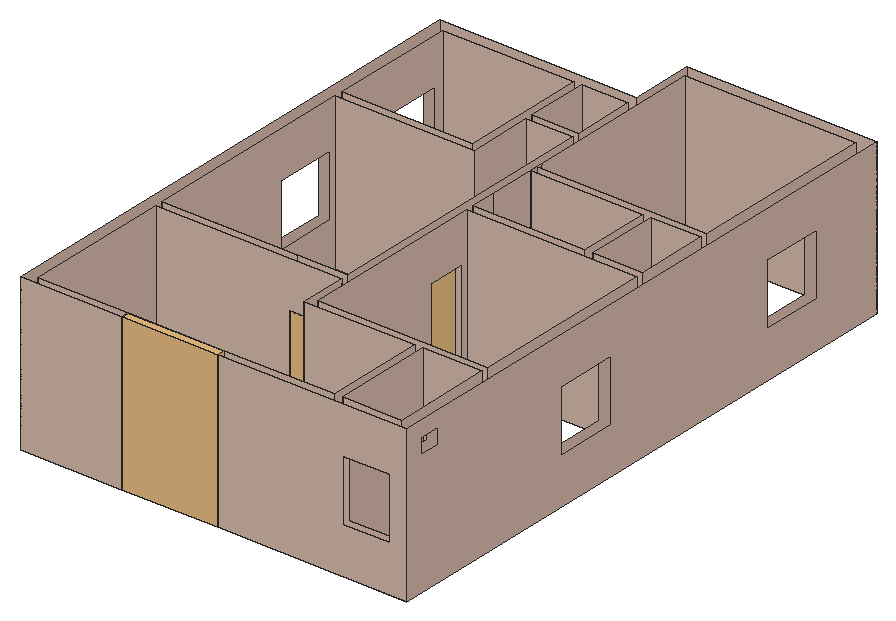
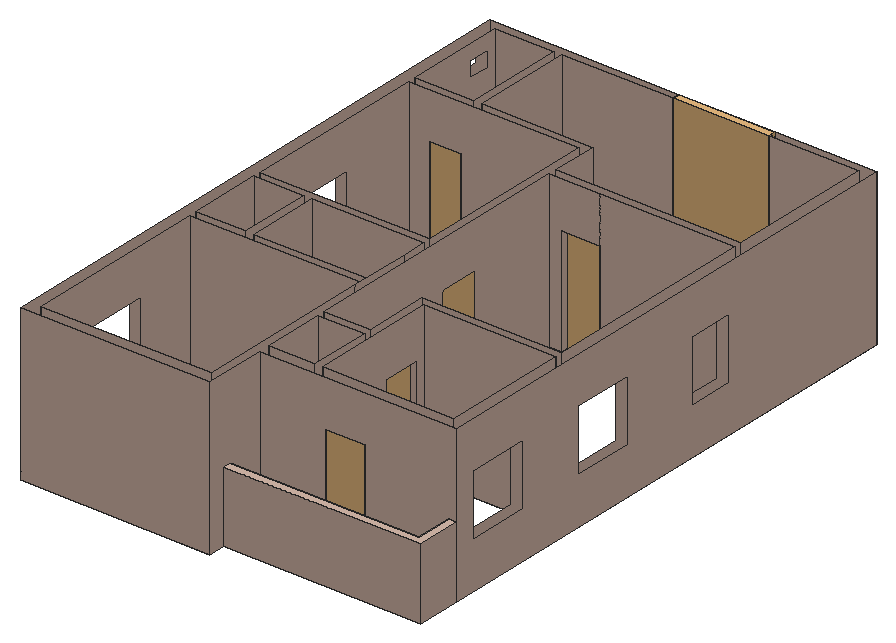
# SketchUp Ruby script. Lengths in inches.
U = 1.inch
M = Sketchup.active_model
def pt(a) = Geom::Point3d.new(a.map { |v| v * U })
def face(e, loops, mat)
  f = e.add_face(loops[0].map { |a| pt(a) })
  loops[1..].each { |l| e.add_face(l.map { |a| pt(a) }).erase! }
  f.material = f.back_material = mat if mat
  f
end
# faces: each face lists its corners as indices into pts; further lists are holes
def faces(e, pts, list, mat = nil) = list.each { |f| face(e, (f[0].is_a?(Array) ? f : [f]).map { |l| l.map { |i| pts[i] } }, mat) }
# xy, xz, yz: faces in a plane at the given z, y or x. An outline is a flat list of corners, or four numbers for a rectangle; further outlines are holes
def ring(l) = l.size == 4 ? [[l[0], l[1]], [l[2], l[1]], [l[2], l[3]], [l[0], l[3]]] : l.each_slice(2).to_a
def flat(e, list, mat, &to3) = list.each { |f| face(e, (f[0].is_a?(Array) ? f : [f]).map { |l| ring(l).map { |u, v| to3.(u, v) } }, mat) }
def xy(e, z, list, mat = nil) = flat(e, list, mat) { |x, y| [x, y, z] }
def xz(e, y, list, mat = nil) = flat(e, list, mat) { |x, z| [x, y, z] }
def yz(e, x, list, mat = nil) = flat(e, list, mat) { |y, z| [x, y, z] }
def lines(e, pts, list) = list.each { |a, b| e.add_line(pt(pts[a]), pt(pts[b])) }
# prism: a flat outline (further loops are holes) pulled along v
def prism(e, loops, v, mat = nil)
  f = face(e, loops, mat); d = Geom::Vector3d.new(v.map { |x| x * U })
  f.pushpull(f.normal.samedirection?(d) ? d.length : -d.length)
end
def box(e, o, s, mat = nil) = prism(e, [[o, [o[0] + s[0], o[1], o[2]], [o[0] + s[0], o[1] + s[1], o[2]], [o[0], o[1] + s[1], o[2]]]], [0, 0, s[2]], mat)
def at(x, y, z, deg = 0) = Geom::Transformation.translation(pt([x, y, z])) * Geom::Transformation.rotation(ORIGIN, Z_AXIS, deg.degrees)
def axes(o, x, y, z) = Geom::Transformation.new([*x, 0, *y, 0, *z, 0, *pt(o).to_a, 1])
def part(name) = M.definitions.add(name)
# library, detail: a bought-in or finely detailed component or shape, given as its bounding box
def library(name, o, s) = part(name).tap { |d| box(d.entities, o, s) }
def detail(e, o, s) = box(e.add_group.entities, o, s)
def put(e, d, t, mat = nil) = e.add_instance(d, t).tap { |i| i.material = mat if mat }
def group(e, t, mat = nil) = e.add_group.tap { |g| g.transformation = t; g.material = mat if mat }.entities
root = M.entities
M.materials.add("[Color B01]").color = [216, 187, 172]
M.materials.add("[Wood Cherry Original]").color = [152, 86, 42]
c1 = library("Sliding Door (1.93 x 2.21)",[0,-1.25,-0.01],[76.06,6.25,87.01])
c2 = library("door by lz",[5.91,-4.92,0],[35.43,6.61,78.74])
c3 = part("Union\#3")
prism(c3.entities,[[[153,29,0],[6,29,0],[6,0,0],[0,0,0],[0,35,0],[153,35,0]]],[0,0,55.4375])
xy(root,155.75,[[0,134.5,0,541.5,71.05,541.5,71.05,532.5,9,532.5,9,434.5,117,434.5,117,428.5,9,428.5,9,260.5,113.3,260.5,113.3,254.5,9,254.5,9,140.5,78.6875,140.5,78.6875,134.5],[[153,134.5,153,140.5,239,140.5,239,218.5,153,218.5,153,254.5,143.3,254.5,143.3,260.5,153,260.5,153,333.45,159,333.45,159,224.5,250.23,224.5,250.23,218.5,245,218.5,245,140.5,291,140.5,291,218.5,274.23,218.5,274.23,224.5,291,224.5,291,368.5,159,368.5,159,363.45,153,363.45,153,394.3125,159,394.3125,159,374.5,246,374.5,246,430.5,159,430.5,159,436.5,291,436.5,291,580.5,159,580.5,159,471.27,153,471.27,153,478.5,144.37,478.5,144.37,484.5,153,484.5,153,532.5,117,532.5,117,484.5,124.37,484.5,124.37,478.5,117,478.5,117,471.23,111,471.23,111,532.5,101.05,532.5,101.05,541.5,153,541.5,153,589.5,300,589.5,300,134.5],[252,374.5,291,430.5]],[153,424.3125,158.97,441.27],[111,434.5,117,441.27]],"[Color B01]")
xz(root,134.5,[[0,155.75,78.6875,275.75],[[153,155.75,300,275.75],[250.39,191.75,286.39,239.75]]],"[Color B01]")
xz(root,140.5,[[9,155.75,78.6875,275.75],[153,155.75,239,275.75],[[245,155.75,291,275.75],[250.39,191.75,286.39,239.75]]],"[Color B01]")
xz(root,218.5,[[153,155.75,239,275.75],[245,155.75,250.23,155.75,250.23,239.75,274.23,239.75,274.23,155.75,291,155.75,291,275.75,245,275.75]],"[Color B01]")
xz(root,224.5,[[159,155.75,159,275.75,291,275.75,291,155.75,274.23,155.75,274.23,239.75,250.23,239.75,250.23,155.75]],"[Color B01]")
xz(root,254.5,[[9,155.75,113.3,155.75,113.3,239.75,143.3,239.75,143.3,155.75,153,155.75,153,275.75,9,275.75]],"[Color B01]")
xz(root,260.5,[[9,155.75,113.3,275.75],[143.3,155.75,143.3,239.75,113.3,239.75,113.3,275.75,153,275.75,153,155.75]],"[Color B01]")
xz(root,333.45,[[153,155.75,159,239.75]],"[Color B01]")
xz(root,363.45,[[153,155.75,159,239.75]],"[Color B01]")
xz(root,368.5,[[159,155.75,291,275.75]],"[Color B01]")
xz(root,374.5,[[159,155.75,246,275.75],[252,155.75,291,275.75]],"[Color B01]")
xz(root,394.3125,[[153,155.75,153,239.75,158.97,239.75,158.97,275.75,159,275.75,159,155.75]],"[Color B01]")
xz(root,424.3125,[[153,155.75,158.97,239.75]],"[Color B01]")
xz(root,428.5,[[9,155.75,117,275.75]],"[Color B01]")
xz(root,430.5,[[159,155.75,246,275.75],[252,155.75,291,275.75]],"[Color B01]")
xz(root,434.5,[[9,155.75,111,275.75]],"[Color B01]")
xz(root,436.5,[[159,155.75,291,275.75]],"[Color B01]")
xz(root,441.27,[[111,155.75,117,239.75],[153,155.75,158.97,239.75]],"[Color B01]")
xz(root,471.23,[[111,155.75,117,239.75]],"[Color B01]")
xz(root,471.27,[[153,155.75,159,239.75]],"[Color B01]")
xz(root,478.5,[[117,155.75,124.37,155.75,124.37,239.75,144.37,239.75,144.37,155.75,153,155.75,153,275.75,117,275.75]],"[Color B01]")
xz(root,484.5,[[117,155.75,117,275.75,153,275.75,153,155.75,144.37,155.75,144.37,239.75,124.37,239.75,124.37,155.75]],"[Color B01]")
xz(root,532.5,[[9,155.75,71.05,155.75,71.05,239.75,101.05,239.75,101.05,155.75,111,155.75,111,275.75,9,275.75],[117,155.75,153,275.75]],"[Color B01]")
xz(root,541.5,[[0,155.75,0,275.75,153,275.75,153,155.75,101.05,155.75,101.05,239.75,71.05,239.75,71.05,155.75]],"[Color B01]")
xz(root,580.5,[[159,155.75,291,275.75]],"[Color B01]")
xz(root,589.5,[[153,155.75,300,275.75]],"[Color B01]")
yz(root,0,[[[134.5,155.75,541.5,275.75],[477.49,191.75,525.49,239.75],[375.61,191.75,423.61,239.75],[277.6875,191.75,313.6875,239.75]]],"[Color B01]")
yz(root,9,[[140.5,155.75,254.5,275.75],[[260.5,155.75,428.5,275.75],[375.61,191.75,423.61,239.75],[277.6875,191.75,313.6875,239.75]],[[434.5,155.75,532.5,275.75],[477.49,191.75,525.49,239.75]]],"[Color B01]")
yz(root,71.05,[[532.5,155.75,541.5,239.75]],"[Color B01]")
yz(root,78.6875,[[134.5,155.75,140.5,275.75]],"[Color B01]")
yz(root,101.05,[[532.5,155.75,541.5,239.75]],"[Color B01]")
yz(root,111,[[434.5,155.75,434.5,275.75,532.5,275.75,532.5,155.75,471.23,155.75,471.23,239.75,441.27,239.75,441.27,155.75]],"[Color B01]")
yz(root,113.3,[[254.5,155.75,260.5,239.75]],"[Color B01]")
yz(root,117,[[428.5,155.75,441.27,155.75,441.27,239.75,471.23,239.75,471.23,155.75,478.5,155.75,478.5,275.75,428.5,275.75],[484.5,155.75,532.5,275.75]],"[Color B01]")
yz(root,124.37,[[478.5,155.75,484.5,239.75]],"[Color B01]")
yz(root,143.3,[[254.5,155.75,260.5,239.75]],"[Color B01]")
yz(root,144.37,[[478.5,155.75,484.5,239.75]],"[Color B01]")
yz(root,153,[[134.5,155.75,140.5,275.75],[218.5,155.75,254.5,275.75],[260.5,155.75,260.5,275.75,478.5,275.75,478.5,155.75,471.27,155.75,471.27,239.75,441.27,239.75,441.27,155.75,424.3125,155.75,424.3125,239.75,394.3125,239.75,394.3125,155.75,363.45,155.75,363.45,239.75,333.45,239.75,333.45,155.75],[484.5,155.75,532.5,275.75],[541.5,155.75,589.5,275.75]],"[Color B01]")
yz(root,158.97,[[424.3125,155.75,441.27,155.75,441.27,275.75,394.3125,275.75,394.3125,239.75,424.3125,239.75]],"[Color B01]")
yz(root,159,[[224.5,155.75,333.45,155.75,333.45,239.75,363.45,239.75,363.45,155.75,368.5,155.75,368.5,275.75,224.5,275.75],[374.5,155.75,394.3125,275.75],[430.5,155.75,436.5,275.75],[471.27,155.75,580.5,155.75,580.5,275.75,441.27,275.75,441.27,239.75,471.27,239.75]],"[Color B01]")
yz(root,239,[[140.5,155.75,218.5,275.75]],"[Color B01]")
yz(root,245,[[140.5,155.75,218.5,275.75]],"[Color B01]")
yz(root,246,[[374.5,155.75,430.5,275.75]],"[Color B01]")
yz(root,250.23,[[218.5,155.75,224.5,239.75]],"[Color B01]")
yz(root,252,[[374.5,155.75,430.5,275.75]],"[Color B01]")
yz(root,274.23,[[218.5,155.75,224.5,239.75]],"[Color B01]")
yz(root,291,[[[140.5,155.75,218.5,275.75],[147.54,251.75,164.47,263.75]],[[224.5,155.75,368.5,275.75],[283.77,191.75,331.77,239.75]],[374.5,155.75,430.5,275.75],[[436.5,155.75,580.5,275.75],[483.51,191.75,531.51,239.75]]],"[Color B01]")
yz(root,300,[[[134.5,155.75,589.5,275.75],[483.51,191.75,531.51,239.75],[283.77,191.75,331.77,239.75],[147.54,251.75,164.47,263.75]]],"[Color B01]")
put(root,c1,axes([78.6875,135.75,155.75],[0.97705,0,0],[0,1,0],[0,0,1.37927]),"[Wood Cherry Original]")
put(root,c2,axes([108.3,255.09,155.75],[0.84667,0,0],[0,0.14881,0],[0,0,1.0668]),"[Color B01]")
put(root,c2,axes([66.05,541.59,155.75],[0.84667,0,0],[0,0.14881,0],[0,0,1.0668]),"[Color B01]")
put(root,c3,at(0,541.5,155.75),"[Color B01]")
put(root,c2,axes([153.59,476.27,155.75],[0,-0.84667,0],[0.14881,0,0],[0,0,1.0668]),"[Color B01]")
put(root,c2,axes([153.59,368.46,155.75],[0,-0.84667,0],[0.14881,0,0],[0,0,1.0668]),"[Color B01]")
put(root,c2,axes([153.59,429.32,155.75],[0,-0.84667,0],[0.14881,0,0],[0,0,1.0668]),"[Color B01]")
put(root,c2,axes([116.41,476.27,155.75],[0,-0.84667,0],[-0.14881,0,0],[0,0,1.0668]),"[Color B01]")
put(root,c2,axes([246.23,224.5,155.75],[0.67733,0,0],[0,0.14881,0],[0,0,1.0668]),"[Color B01]")
